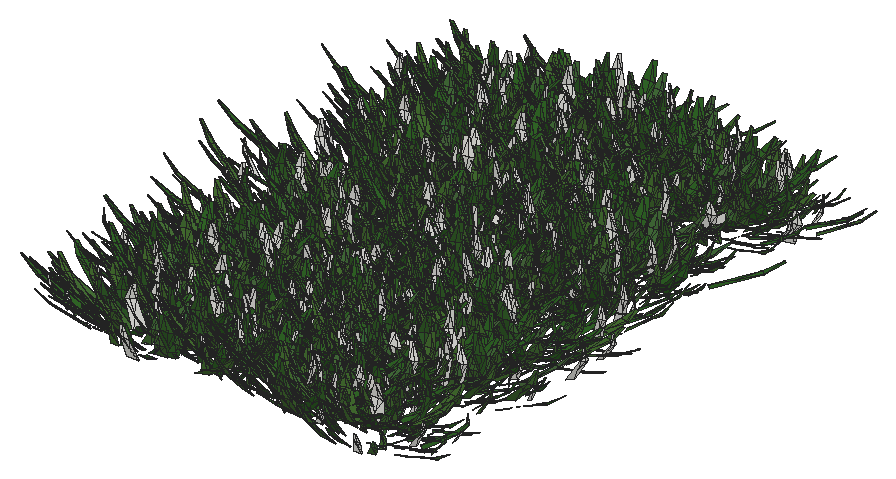
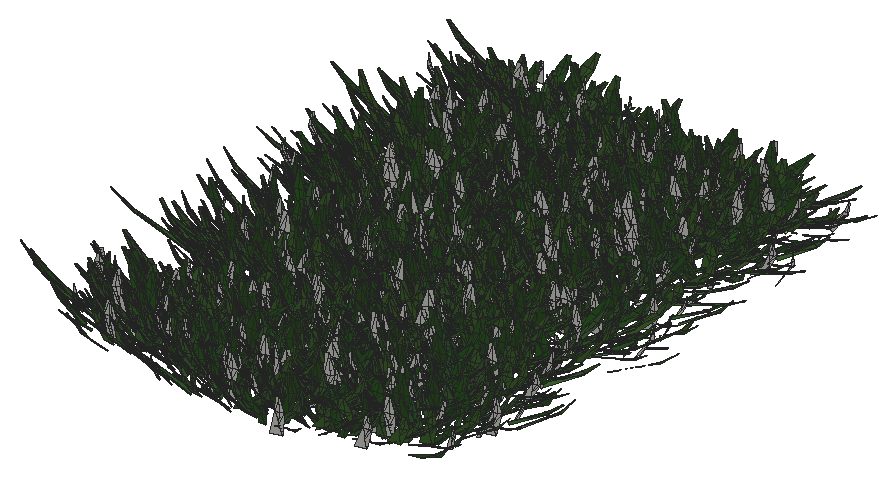
# SketchUp Ruby script. Lengths in inches.
U = 1.inch
M = Sketchup.active_model
def pt(a) = Geom::Point3d.new(a.map { |v| v * U })
def face(e, loops, mat)
  f = e.add_face(loops[0].map { |a| pt(a) })
  loops[1..].each { |l| e.add_face(l.map { |a| pt(a) }).erase! }
  f.material = f.back_material = mat if mat
  f
end
# faces: each face lists its corners as indices into pts; further lists are holes
def faces(e, pts, list, mat = nil) = list.each { |f| face(e, (f[0].is_a?(Array) ? f : [f]).map { |l| l.map { |i| pts[i] } }, mat) }
# xy, xz, yz: faces in a plane at the given z, y or x. An outline is a flat list of corners, or four numbers for a rectangle; further outlines are holes
def ring(l) = l.size == 4 ? [[l[0], l[1]], [l[2], l[1]], [l[2], l[3]], [l[0], l[3]]] : l.each_slice(2).to_a
def flat(e, list, mat, &to3) = list.each { |f| face(e, (f[0].is_a?(Array) ? f : [f]).map { |l| ring(l).map { |u, v| to3.(u, v) } }, mat) }
def xy(e, z, list, mat = nil) = flat(e, list, mat) { |x, y| [x, y, z] }
def xz(e, y, list, mat = nil) = flat(e, list, mat) { |x, z| [x, y, z] }
def yz(e, x, list, mat = nil) = flat(e, list, mat) { |y, z| [x, y, z] }
def lines(e, pts, list) = list.each { |a, b| e.add_line(pt(pts[a]), pt(pts[b])) }
# prism: a flat outline (further loops are holes) pulled along v
def prism(e, loops, v, mat = nil)
  f = face(e, loops, mat); d = Geom::Vector3d.new(v.map { |x| x * U })
  f.pushpull(f.normal.samedirection?(d) ? d.length : -d.length)
end
def box(e, o, s, mat = nil) = prism(e, [[o, [o[0] + s[0], o[1], o[2]], [o[0] + s[0], o[1] + s[1], o[2]], [o[0], o[1] + s[1], o[2]]]], [0, 0, s[2]], mat)
def at(x, y, z, deg = 0) = Geom::Transformation.translation(pt([x, y, z])) * Geom::Transformation.rotation(ORIGIN, Z_AXIS, deg.degrees)
def axes(o, x, y, z) = Geom::Transformation.new([*x, 0, *y, 0, *z, 0, *pt(o).to_a, 1])
def part(name) = M.definitions.add(name)
# library, detail: a bought-in or finely detailed component or shape, given as its bounding box
def library(name, o, s) = part(name).tap { |d| box(d.entities, o, s) }
def detail(e, o, s) = box(e.add_group.entities, o, s)
def put(e, d, t, mat = nil) = e.add_instance(d, t).tap { |i| i.material = mat if mat }
def group(e, t, mat = nil) = e.add_group.tap { |g| g.transformation = t; g.material = mat if mat }.entities
root = M.entities
M.materials.add("Material82").color = [68, 110, 58]
M.materials.add("Material83").color = [48, 90, 38]
M.materials.add("Material84").color = [68, 110, 48]
M.materials.add("Material85").color = [48, 90, 48]
M.materials.add("Material86").color = [58, 110, 58]
M.materials.add("Material87").color = [58, 90, 38]
M.materials.add("Material88").color = [68, 100, 58]
M.materials.add("Material89").color = [48, 100, 38]
c1 = part("grass00")
p = [[-0.6875,0.15,0],[-0.56,0.08,5.52],[-0.04,0.03,2.76],[0.48,-0.02,0],[0.35,-0.02,5.52],[-0.1,-0.14,5.52],
  [-0.12,0.65,8.37],[-0.42,0.65,8.37]]
faces(c1.entities,p,[[0,1,2,3],[3,2,4],[1,5,2],[5,4,2],[1,6,5],[4,5,6],[7,6,1]])
c2 = part("Group16\#1")
put(c2.entities,c1,axes([1.44,-0.61,-0.01],[0.05352,0.12609,0],[-0.10704,0.04543,0.07239],[0.06664,-0.02828,0.11628]),"Material85")
put(c2.entities,c1,axes([0.76,-0.15,-0.01],[0.04676,0.24062,0],[-0.23162,0.04501,0.06642],[0.0652,-0.01267,0.23595]),"Material82")
put(c2.entities,c1,axes([0.79,0.01,-0.01],[-0.00606,0.34651,0],[-0.34381,-0.00602,0.0432],[0.04319,0.00076,0.34386]))
put(c2.entities,c1,axes([1,0.23,-0.01],[-0.07192,0.31144,0],[-0.28722,-0.06632,0.1236],[0.12043,0.02781,0.29478]),"Material84")
put(c2.entities,c1,axes([1.66,0.77,-0.01],[-0.13828,0.29651,0],[-0.21551,-0.1005,0.22471],[0.20365,0.09498,0.23779]),"Material89")
put(c2.entities,c1,axes([0.6875,0.52,-0.01],[-0.18126,0.24051,0],[-0.22746,-0.17142,0.09788],[0.07817,0.05891,0.28481]),"Material84")
put(c2.entities,c1,axes([0.68,0.78,-0.01],[-0.215,0.18688,0],[-0.12385,-0.14248,0.21334],[0.13995,0.16101,0.18878]),"Material82")
put(c2.entities,c1,axes([0.56,1,-0.01],[-0.13756,0.07624,0],[-0.06159,-0.11112,0.0927],[0.04494,0.08108,0.12705]),"Material84")
put(c2.entities,c1,axes([0.2,0.64,-0.01],[-0.23729,0.07254,0],[-0.05711,-0.18681,0.153],[0.04473,0.14632,0.19535]),"Material89")
put(c2.entities,c1,axes([0.0625,0.72,-0.01],[-0.28874,0.02525,0],[-0.02179,-0.24916,0.14647],[0.01276,0.14591,0.25012]),"Material82")
put(c2.entities,c1,axes([-0.08,0.62,-0.01],[-0.34089,-0.04187,0],[0.03255,-0.26504,0.216],[-0.02633,0.21439,0.26703]),"Material89")
put(c2.entities,c1,axes([-0.34,0.98,-0.01],[-0.14314,-0.0493,0],[0.04397,-0.12769,0.06843],[-0.02228,0.0647,0.13505]),"Material89")
put(c2.entities,c1,axes([-0.87,1.45,-0.01],[-0.23488,-0.14114,0],[0.13761,-0.22901,0.06087],[-0.03135,0.05217,0.26717]))
put(c2.entities,c1,axes([-0.72,0.77,-0.01],[-0.14208,-0.13251,0],[0.07209,-0.0773,0.16301],[-0.11118,0.11922,0.1057]),"Material89")
put(c2.entities,c1,axes([-0.62,0.43,-0.01],[-0.14845,-0.21203,0],[0.18654,-0.13061,0.12304],[-0.10079,0.07057,0.22772]),"Material82")
put(c2.entities,c1,axes([-0.68,0.29,-0.01],[-0.13639,-0.32136,0],[0.31723,-0.13464,0.05579],[-0.05136,0.0218,0.34462]),"Material83")
put(c2.entities,c1,axes([-0.64,0.125,-0.01],[-0.0458,-0.23569,0],[0.22124,-0.043,0.08276],[-0.08124,0.01579,0.22538]),"Material86")
put(c2.entities,c1,axes([-1.6,-0.03,-0.01],[0.00576,-0.32897,0],[0.27526,0.00482,0.18018],[-0.18015,-0.00315,0.2753]),"Material84")
put(c2.entities,c1,axes([-1.36,-0.31,-0.01],[0.05718,-0.24765,0],[0.18172,0.04196,0.17267],[-0.16825,-0.03885,0.1865]),"Material89")
put(c2.entities,c1,axes([-1.54,-0.72,-0.01],[0.06537,-0.14017,0],[0.13555,0.06321,0.03939],[-0.0357,-0.01665,0.14956]))
put(c2.entities,c1,axes([-1.19,-0.9,-0.01],[0.09597,-0.12735,0],[0.11214,0.08451,0.07557],[-0.06035,-0.04548,0.14042]),"Material88")
put(c2.entities,c1,axes([-0.47,-0.54,-0.01],[0.11588,-0.10072,0],[0.0618,0.0711,0.12124],[-0.07953,-0.0915,0.0942]))
put(c2.entities,c1,axes([-0.47,-0.84,-0.01],[0.11927,-0.0661,0],[0.06603,0.11913,0.00646],[-0.00313,-0.00565,0.13621]),"Material84")
put(c2.entities,c1,axes([-0.38,-1.24,-0.01],[0.28037,-0.08571,0],[0.0618,0.20215,0.20315],[-0.05939,-0.19428,0.21139]),"Material88")
put(c2.entities,c1,axes([-0.06,-0.66,-0.01],[0.22719,-0.01987,0],[0.01247,0.14255,0.17758],[-0.01547,-0.17691,0.1431]),"Material87")
put(c2.entities,c1,axes([0.11,-0.89,-0.01],[0.14882,0.01828,0],[-0.01058,0.08611,0.12229],[0.01491,-0.12138,0.08676]),"Material85")
put(c2.entities,c1,axes([0.25,-0.72,-0.01],[0.20481,0.07053,0],[-0.06206,0.18022,0.10291],[0.03351,-0.0973,0.1906]),"Material85")
put(c2.entities,c1,axes([0.85,-1.42,-0.01],[0.16481,0.09904,0],[-0.09472,0.15762,0.05616],[0.02893,-0.04814,0.18389]),"Material84")
put(c2.entities,c1,axes([1.01,-1.09,-0.01],[0.21858,0.20385,0],[-0.17495,0.1876,0.15339],[0.10462,-0.11218,0.25652]),"Material89")
put(c2.entities,c1,axes([1.01,-0.71,-0.01],[0.08733,0.12473,0],[-0.06445,0.04512,0.13037],[0.1068,-0.07477,0.07867]),"Material85")
c3 = part("Group15\#1")
put(c3.entities,c2,at(0,0,0))
c4 = part("3darcstudiotree_grass00\#1")
put(c4.entities,c3,at(0,0,0))
put(root,c4,axes([1764.47,953.26,-29.74],[1.08587,1.67228,0],[-4.264,0.43062,-0.00469],[-0.02209,0.00223,1.60422]))
put(root,c4,axes([1765.97,973.1875,-29.74],[-3.39635,0.60304,0],[-1.8174,-1.59194,-0.05685],[-0.1325,-0.11606,1.88376]))
put(root,c4,axes([1765.31,943.77,-29.74],[-0.8053,1.43922,0],[-4.1788,-0.36366,-0.05256],[-0.20936,-0.01822,1.30827]))
put(root,c4,axes([1766.12,990.89,-29.74],[1.7154,-1.15643,0],[3.09768,0.71465,-0.02347],[0.14538,0.03354,1.9305]))
put(root,c4,axes([1766.8,971.14,-29.74],[-0.55616,-1.38612,0],[4.6364,-0.28933,-0.05346],[0.22148,-0.01382,1.47567]))
put(root,c4,axes([1766.16,949.59,-29.74],[2.313,-1.43442,0],[2.99954,0.75225,-0.04064],[0.1888,0.04735,1.46692]))
put(root,c4,axes([1766.23,988.37,-29.74],[2.50193,-0.87133,0],[2.32937,1.04026,-0.01409],[0.05813,0.02596,1.64399]))
put(root,c4,axes([1766.46,958.98,-29.74],[2.27709,-1.12887,0],[2.96357,0.92974,-0.01848],[0.07518,0.02359,1.47553]))
put(root,c4,axes([1765.4,986.68,-29.74],[4.07348,0.57799,0],[-1.18057,1.29405,-0.01256],[-0.02962,0.03247,1.82155]))
put(root,c4,axes([1765.55,969.1,-29.74],[2.25028,1.20461,0],[-3.26486,0.94856,-0.0323],[-0.12798,0.03718,1.496]))
put(root,c4,axes([1766.18,980.93,-29.74],[-1.39977,1.36626,0],[-3.55438,-0.56636,-0.02451],[-0.1313,-0.02092,1.66036]))
put(root,c4,axes([1765.67,950.59,-29.74],[3.43029,0.99275,0],[-1.97308,1.06035,-0.01519],[-0.04853,0.02608,1.34969]))
put(root,c4,axes([1766.625,946.78,-29.74],[-1.21632,1.56365,0],[-3.36368,-0.40694,-0.03727],[-0.21338,-0.02582,1.57911]))
put(root,c4,axes([1766,963.77,-29.74],[4.01997,0.45296,0],[-1.05214,1.45226,-0.01128],[-0.01738,0.02399,1.61003]))
put(root,c4,axes([1766.32,966.45,-29.74],[4.2861,-0.44175,0],[0.90749,1.36943,-0.02428],[0.0455,0.06867,1.99391]))
put(root,c4,axes([1766.625,983.88,-29.74],[3.51248,0.23364,0],[-0.65189,1.52422,-0.03005],[-0.02625,0.06139,1.54341]))
put(root,c4,axes([1767.13,942.05,-29.74],[3.31562,-0.63662,0],[1.81859,1.47309,-0.02466],[0.05194,0.04207,1.49812]))
put(root,c4,axes([1767.43,977.47,-29.74],[-0.84571,1.33613,0],[-3.59715,-0.35412,-0.00012],[-0.00056,-0.00006,1.39497]))
put(root,c4,axes([1767.76,992.93,-29.74],[-1.51727,1.49458,0],[-3.30202,-0.52136,-0.01826],[-0.09361,-0.01478,1.47196]))
put(root,c4,axes([1768.125,955.89,-29.74],[3.22727,-0.96219,0],[2.40393,1.25403,-0.04167],[0.15655,0.08166,1.86151]))
put(root,c4,axes([1769.59,953.09,-29.74],[-3.43052,-0.93956,0],[2.00829,-1.14045,-0.00375],[0.01479,-0.0084,1.82358]))
put(root,c4,axes([1769.65,946.7,-29.74],[-2.79747,-0.82267,0],[2.4,-1.26929,-0.00029],[0.00098,-0.00052,1.69542]))
put(root,c4,axes([1768.03,980.14,-29.74],[3.76479,0.94059,0],[-2.16386,1.34705,-0.03414],[-0.08584,0.05343,1.42377]))
put(root,c4,axes([1769.74,960.45,-29.74],[-3.74102,0.70585,0],[-1.92999,-1.5909,-0.05113],[-0.08819,-0.0727,1.33965]))
put(root,c4,axes([1770.01,982.32,-29.74],[2.94171,-1.11183,0],[3.18535,1.31078,-0.03986],[0.13301,0.05473,1.66404]))
put(root,c4,axes([1770.49,941.6875,-29.74],[-3.65106,0.9561,0],[-2.55118,-1.5152,-0.05111],[-0.12576,-0.07469,1.53759]))
put(root,c4,axes([1770.46,968.48,-29.74],[-2.1448,1.18286,0],[-3.37437,-0.95161,-0.05929],[-0.21963,-0.06194,1.41608]))
put(root,c4,axes([1769.625,951.12,-29.74],[2.61816,1.29298,0],[-2.60516,0.82044,-0.01421],[-0.06264,0.01973,1.40932]))
put(root,c4,axes([1771.41,983.85,-29.74],[-0.23596,-1.70659,0],[3.32039,-0.0714,-0.01049],[0.06174,-0.00133,1.4693]))
put(root,c4,axes([1772.3125,985.85,-29.74],[-2.68837,-0.8629,0],[2.90522,-1.40773,-0.04334],[0.1065,-0.05161,1.34295]))
put(root,c4,axes([1771.64,980.02,-29.74],[2.30193,-1.12166,0],[3.41965,1.0915,-0.0352],[0.15447,0.0493,1.86157]))
put(root,c4,axes([1772.61,977.03,-29.74],[-3.8851,-1.03716,0],[2.44189,-1.42264,-0.04034],[0.11257,-0.06558,1.62559]))
put(root,c4,axes([1770.54,957.93,-29.74],[4.25337,0.6683,0],[-1.56461,1.54873,-0.01606],[-0.02903,0.02874,1.54782]))
put(root,c4,axes([1770.84,975.2,-29.74],[0.91536,1.26151,0],[-4.37209,0.4934,-0.02742],[-0.14974,0.0169,1.93645]))
put(root,c4,axes([1771.09,966.12,-29.74],[-0.09975,1.34747,0],[-4.08432,-0.04703,-0.00454],[-0.02466,-0.00028,1.66362]))
put(root,c4,axes([1773.08,964.17,-29.74],[-1.28823,-1.73919,0],[3.44626,-0.39701,-0.03009],[0.18497,-0.02131,1.72353]))
put(root,c4,axes([1771.98,995.19,-29.74],[3.82297,0.44431,0],[-0.93883,1.25636,-0.026],[-0.04711,0.06304,1.59572]))
put(root,c4,axes([1773.51,991.98,-29.74],[1.61408,-1.6002,0],[4.35972,0.68394,-0.04298],[0.19186,0.0301,1.68954]))
put(root,c4,axes([1772.17,989.56,-29.74],[4.08766,0.51132,0],[-1.24704,1.55051,-0.00141],[-0.00269,0.00335,1.95289]))
put(root,c4,axes([1772.65,944.97,-29.74],[0.40934,1.39565,0],[-3.638,0.16595,-0.04522],[-0.26335,0.01201,1.60941]))
put(root,c4,axes([1773.06,949.33,-29.74],[-2.97215,1.15542,0],[-3.15373,-1.26173,-0.01243],[-0.04576,-0.01831,1.76595]))
put(root,c4,axes([1773.07,987.72,-29.74],[4.03922,-0.03156,0],[0.07296,1.45219,-0.01855],[0.00258,0.0513,1.93628]))
put(root,c4,axes([1773.16,955.45,-29.74],[1.39622,1.62786,0],[-3.6301,0.48424,-0.04556],[-0.23124,0.03085,1.53888]))
put(root,c4,axes([1773.66,961.14,-29.74],[4.28281,-0.63976,0],[1.42181,1.48036,-0.01068],[0.01649,0.01717,1.31138]))
put(root,c4,axes([1773.62,973.6,-29.74],[3.35774,0.54146,0],[-1.57719,1.52117,-0.03911],[-0.07127,0.06874,1.50402]))
put(root,c4,axes([1775.55,964.76,-29.74],[-1.97401,-1.44609,0],[3.51216,-0.74566,-0.02018],[0.11603,-0.02463,1.95264]))
put(root,c4,axes([1775.49,979.34,-29.74],[-2.39621,-0.97294,0],[2.61152,-1.00033,-0.02073],[0.08443,-0.03234,1.5494]))
put(root,c4,axes([1773.54,970.62,-29.74],[2.01516,1.65729,0],[-3.55056,0.67146,-0.00104],[-0.005,0.00095,1.58037]))
put(root,c4,axes([1776.04,976.84,-29.74],[-3.41262,-0.98405,0],[2.00346,-1.0806,-0.03203],[0.14502,-0.07822,1.95145]))
put(root,c4,axes([1775.22,942.67,-29.74],[3.35024,-0.43777,0],[1.10858,1.31952,-0.03222],[0.06859,0.08164,1.78787]))
put(root,c4,axes([1775.86,994.33,-29.74],[2.23301,-1.20393,0],[2.80312,0.80861,-0.02877],[0.133,0.03837,1.49076]))
put(root,c4,axes([1777.32,973.25,-29.74],[-1.89614,-1.52378,0],[3.69892,-0.71587,-0.01008],[0.04587,-0.00888,1.566]))
put(root,c4,axes([1775.73,946.05,-29.74],[0.10079,1.33733,0],[-4.05045,0.04748,-0.05613],[-0.28184,0.0033,1.5259]))
put(root,c4,axes([1776.44,967.75,-29.74],[3.01451,-0.88182,0],[2.30556,1.22582,-0.02804],[0.08966,0.04767,1.55696]))
put(root,c4,axes([1775.67,945.2,-29.74],[2.52987,0.96809,0],[-2.35442,0.95693,-0.00683],[-0.03278,0.01332,1.74693]))
put(root,c4,axes([1777.19,990.53,-29.74],[-4.40755,0.3662,0],[-0.80873,-1.51388,-0.00142],[-0.00162,-0.00303,1.63114]))
put(root,c4,axes([1777.46,970.07,-29.74],[-3.86461,-0.59074,0],[1.45311,-1.4785,-0.05586],[0.12869,-0.13094,1.92103]))
put(root,c4,axes([1777.59,954.54,-29.74],[0.04452,-1.40138,0],[3.5701,0.01764,-0.00992],[0.04898,0.00024,1.32167]))
put(root,c4,axes([1777.3125,992.66,-29.74],[-3.74567,1.07998,0],[-2.52019,-1.35944,-0.03994],[-0.14532,-0.07839,1.97331]))
put(root,c4,axes([1776.27,985.13,-29.74],[4.59378,0.22046,0],[-0.54654,1.77125,-0.0359],[-0.02405,0.07793,1.88046]))
put(root,c4,axes([1777.61,980.81,-29.74],[1.47145,-1.32607,0],[3.01918,0.52105,-0.00213],[0.01031,0.00178,1.30651]))
put(root,c4,axes([1778.73,948.32,-29.74],[-2.64283,-1.13535,0],[3.48014,-1.25993,-0.02326],[0.08818,-0.03192,1.82249]))
put(root,c4,axes([1778.1875,951.53,-29.74],[1.26532,-1.44178,0],[3.12553,0.42661,-0.00044],[0.00223,0.0003,1.32507]))
put(root,c4,axes([1778.71,961.61,-29.74],[-4.13794,-0.2249,0],[0.58111,-1.66288,-0.00876],[0.00496,-0.01418,1.32289]))
put(root,c4,axes([1777.75,983.75,-29.74],[-2.89048,1.44179,0],[-2.90546,-0.90593,-0.0043],[-0.02277,-0.0071,1.8735]))
put(root,c4,axes([1776.85,975.54,-29.74],[2.24895,1.38406,0],[-3.92977,0.99312,-0.02786],[-0.13256,0.0335,1.9768]))
put(root,c4,axes([1777.81,952.74,-29.74],[3.40614,0.32781,0],[-0.81542,1.31776,-0.01459],[-0.02356,0.03807,1.75568]))
put(root,c4,axes([1777.88,996.99,-29.74],[4.11101,0.00408,0],[-0.01055,1.6533,-0.01268],[-0.00019,0.02913,1.83013]))
put(root,c4,axes([1778.03,988.6875,-29.74],[4.61322,-0.12203,0],[0.30512,1.79396,-0.00473],[0.00139,0.00815,1.49489]))
put(root,c4,axes([1777.94,957.56,-29.74],[3.60093,0.62069,0],[-1.54425,1.39338,-0.01451],[-0.03218,0.02903,1.59989]))
put(root,c4,axes([1779.04,960.13,-29.74],[-0.93158,1.57452,0],[-3.64716,-0.33561,-0.02125],[-0.09909,-0.00912,1.34411]))
put(root,c4,axes([1778.92,965.66,-29.74],[1.53583,1.49996,0],[-3.93703,0.62697,-0.05886],[-0.22971,0.03658,1.33951]))
put(root,c4,axes([1781.17,959.57,-29.74],[-2.29669,-1.11112,0],[2.95834,-0.95105,-0.00371],[0.01505,-0.00484,1.4993]))
put(root,c4,axes([1781.1,994.95,-29.74],[-2.49297,-0.95003,0],[2.84759,-1.16217,-0.03177],[0.13042,-0.05323,1.8145]))
put(root,c4,axes([1780.91,965.81,-29.74],[-2.8718,1.45727,0],[-2.81901,-0.86401,-0.03149],[-0.12433,-0.03811,1.33797]))
put(root,c4,axes([1780.86,957.45,-29.74],[-2.73949,1.39402,0],[-3.69271,-1.12865,-0.03455],[-0.12332,-0.03769,1.58129]))
put(root,c4,axes([1782.3,985.67,-29.74],[-2.79426,-0.70511,0],[1.77672,-1.09506,-0.02395],[0.07288,-0.04492,1.39534]))
put(root,c4,axes([1781.11,948.12,-29.74],[4.32757,-0.42653,0],[1.12297,1.77206,-0.03338],[0.0321,0.05066,1.37691]))
put(root,c4,axes([1781.38,974.3,-29.74],[3.39282,-0.2362,0],[0.75884,1.6953,-0.03701],[0.03902,0.08718,1.98432]))
put(root,c4,axes([1781.33,983.04,-29.74],[1.01985,1.24994,0],[-3.27441,0.41552,-0.0339],[-0.22651,0.02874,1.80984]))
put(root,c4,axes([1781.78,955.09,-29.74],[3.17214,0.39156,0],[-1.05658,1.33127,-0.01935],[-0.04192,0.05282,1.92273]))
put(root,c4,axes([1782.09,972.06,-29.74],[3.44047,-0.2055,0],[0.68194,1.77564,-0.05863],[0.04271,0.1112,1.66018]))
put(root,c4,axes([1782.9,992.99,-29.74],[-2.53173,1.21264,0],[-2.8931,-0.93942,-0.04557],[-0.23211,-0.07537,1.85346]))
put(root,c4,axes([1783.66,946.88,-29.74],[-3.83423,-0.51133,0],[1.38691,-1.61748,-0.06149],[0.1095,-0.1277,1.80385]))
put(root,c4,axes([1783.76,971.34,-29.74],[-2.06404,-1.37727,0],[3.69374,-0.86095,-0.04139],[0.20463,-0.0477,1.84708]))
put(root,c4,axes([1781.96,981.04,-29.74],[2.13019,1.09948,0],[-3.08878,0.93074,-0.0123],[-0.05365,0.01617,1.59876]))
put(root,c4,axes([1784.04,987.38,-29.74],[-4.29389,-0.13256,0],[0.34176,-1.72178,-0.05117],[0.01874,-0.09441,1.54048]))
put(root,c4,axes([1782.67,942.03,-29.74],[4.09444,0.12503,0],[-0.31641,1.61154,-0.0417],[-0.02006,0.10219,1.91485]))
put(root,c4,axes([1784.03,967.74,-29.74],[-3.97452,0.57658,0],[-1.26948,-1.361,-0.04924],[-0.12234,-0.13116,1.98345]))
put(root,c4,axes([1782.76,979.83,-29.74],[4.64305,-0.03413,0],[0.08366,1.7702,-0.03615],[0.00311,0.0658,1.55355]))
put(root,c4,axes([1782.6,944.35,-29.74],[3.61655,0.77067,0],[-2.16585,1.58076,-0.05913],[-0.11484,0.08382,1.39517]))
put(root,c4,axes([1784.02,950.95,-29.74],[-3.45507,0.18922,0],[-0.60525,-1.7188,-0.02154],[-0.01288,-0.03658,1.4342]))
put(root,c4,axes([1784.41,996.36,-29.74],[-3.18702,-0.48311,0],[1.45771,-1.49562,-0.04802],[0.08757,-0.08985,1.54794]))
put(root,c4,axes([1783.4,952.61,-29.74],[1.33968,1.52005,0],[-3.16755,0.43419,-0.01128],[-0.07711,0.01057,1.81963]))
put(root,c4,axes([1783.97,962.625,-29.74],[-0.83712,1.35251,0],[-3.5635,-0.34303,-0.03757],[-0.17469,-0.01682,1.3158]))
put(root,c4,axes([1784.73,964.89,-29.74],[3.08356,-0.59749,0],[1.85245,1.48689,-0.05746],[0.15906,0.12767,1.97658]))
put(root,c4,axes([1784.62,977.9,-29.74],[1.55645,1.18195,0],[-3.2541,0.66647,-0.04821],[-0.21297,0.04362,1.36797]))
put(root,c4,axes([1784.76,990.47,-29.74],[0.845,1.27042,0],[-4.02841,0.41673,-0.05161],[-0.24313,0.02515,1.52021]))
put(root,c4,axes([1786.95,970.42,-29.74],[-3.70591,-0.99796,0],[1.87776,-1.08451,-0.01838],[0.07513,-0.04339,1.80866]))
put(root,c4,axes([1786.98,986.51,-29.74],[0.0983,-1.39772,0],[3.56781,0.03903,-0.00183],[0.01012,0.00011,1.48199]))
put(root,c4,axes([1786.66,951.6875,-29.74],[2.17735,-1.14497,0],[3.55677,1.05197,-0.03529],[0.11494,0.03399,1.35654]))
put(root,c4,axes([1787.6,964.24,-29.74],[-4.087,-0.33484,0],[0.93219,-1.7696,-0.02537],[0.02744,-0.05209,1.82613]))
put(root,c4,axes([1787.26,975.18,-29.74],[-3.8828,0.51827,0],[-1.09306,-1.27365,-0.02484],[-0.06133,-0.07146,1.96802]))
put(root,c4,axes([1787.54,955.43,-29.74],[-4.01589,0.275,0],[-0.74615,-1.69466,-0.05401],[-0.03733,-0.08478,1.3206]))
put(root,c4,axes([1786.98,960.24,-29.74],[-1.92395,1.11114,0],[-2.73961,-0.73778,-0.01899],[-0.11099,-0.02989,1.75992]))
put(root,c4,axes([1786.32,941.76,-29.74],[-0.14266,1.36173,0],[-4.10184,-0.06683,-0.00296],[-0.01424,-0.00023,1.47961]))
put(root,c4,axes([1786.58,965.58,-29.74],[-0.37072,1.84099,0],[-4.27519,-0.13389,-0.01448],[-0.06545,-0.00205,1.45727]))
put(root,c4,axes([1786.79,994.4,-29.74],[4.18586,0.29447,0],[-0.62505,1.38186,-0.04495],[-0.05854,0.12943,1.97854]))
put(root,c4,axes([1788.87,967.85,-29.74],[-0.69027,-1.34957,0],[4.18043,-0.33255,-0.04603],[0.23408,-0.01862,1.65834]))
put(root,c4,axes([1787.48,943.8,-29.74],[3.68364,0.44666,0],[-1.28613,1.64968,-0.02064],[-0.02718,0.03487,1.46981]))
put(root,c4,axes([1788.82,981.01,-29.74],[-3.79382,0.9598,0],[-2.14839,-1.32076,-0.01729],[-0.051,-0.03135,1.62898]))
put(root,c4,axes([1789.47,952.49,-29.74],[-3.50392,-0.27669,0],[0.88512,-1.7433,-0.02406],[0.02146,-0.04227,1.53532]))
put(root,c4,axes([1789.74,988.08,-29.74],[-4.49069,-0.28234,0],[0.61208,-1.5141,-0.05098],[0.04605,-0.11392,1.67187]))
put(root,c4,axes([1788.29,977.58,-29.74],[4.2001,-0.13479,0],[0.33266,1.61217,-0.01977],[0.00834,0.04041,1.59866]))
put(root,c4,axes([1789.56,979.17,-29.74],[-4.51566,0.3438,0],[-0.75132,-1.53478,-0.00152],[-0.00137,-0.0028,1.41339]))
put(root,c4,axes([1788.5,972,-29.74],[-1.23007,1.60855,0],[-3.72331,-0.44283,-0.01363],[-0.06328,-0.00753,1.41312]))
put(root,c4,axes([1789.1875,946.86,-29.74],[-2.10873,0.99525,0],[-2.92476,-0.96381,-0.03387],[-0.14037,-0.04626,1.54303]))
put(root,c4,axes([1789.03,949.03,-29.74],[3.33633,-0.58263,0],[1.85643,1.65335,-0.04981],[0.10311,0.09183,1.75709]))
put(root,c4,axes([1788.71,983.75,-29.74],[2.36553,1.18037,0],[-3.06807,0.95629,-0.02315],[-0.10187,0.03175,1.64391]))
put(root,c4,axes([1788.59,992.54,-29.74],[2.70315,0.92974,0],[-3.09727,1.40055,-0.01764],[-0.05733,0.02592,1.74631]))
put(root,c4,axes([1789.88,961.79,-29.74],[2.84805,-1.35819,0],[2.78081,0.90692,-0.04304],[0.21584,0.07039,1.76026]))
put(root,c4,axes([1789.33,956.85,-29.74],[0.25957,1.50579,0],[-3.94932,0.10588,-0.02807],[-0.1244,0.00334,1.3177]))
put(root,c4,axes([1791.9375,942.74,-29.74],[-2.56709,-0.87628,0],[2.75862,-1.25691,-0.00422],[0.01164,-0.0053,1.33295]))
put(root,c4,axes([1790.22,990.16,-29.74],[3.46346,0.58344,0],[-1.61207,1.48838,-0.00364],[-0.00911,0.00841,1.96053]))
put(root,c4,axes([1793.0625,988.43,-29.74],[-2.62594,-1.45094,0],[3.42478,-0.964,-0.01802],[0.06257,-0.01761,1.345]))
put(root,c4,axes([1792.57,979.68,-29.74],[-3.57945,0.04189,0],[-0.11544,-1.5341,-0.02538],[-0.0045,-0.05977,1.74242]))
put(root,c4,axes([1791.84,957.48,-29.74],[-2.10864,1.34219,0],[-3.56504,-0.87109,-0.01218],[-0.05259,-0.01285,1.59607]))
put(root,c4,axes([1792.54,951.41,-29.74],[3.4734,-0.75241,0],[2.06047,1.47936,-0.02691],[0.07219,0.05183,1.78778]))
put(root,c4,axes([1793.82,944.38,-29.74],[-1.56362,-1.21345,0],[3.6466,-0.73082,-0.00876],[0.03709,-0.00743,1.45672]))
put(root,c4,axes([1794.05,959.59,-29.74],[-3.17921,-1.35137,0],[3.1644,-1.15784,-0.01209],[0.04457,-0.01631,1.62724]))
put(root,c4,axes([1794.12,963.76,-29.74],[-2.5712,-1.27561,0],[3.33499,-1.0455,-0.01168],[0.0385,-0.01207,1.34439]))
put(root,c4,axes([1792.43,974.79,-29.74],[-0.16089,1.57179,0],[-4.27524,-0.06806,-0.04298],[-0.25282,-0.00402,1.88799]))
put(root,c4,axes([1794.17,968.13,-29.74],[-3.47552,-0.34069,0],[1.08655,-1.72393,-0.01735],[0.02109,-0.03347,1.70162]))
put(root,c4,axes([1794.08,971.25,-29.74],[-3.29266,-0.34854,0],[0.95777,-1.40726,-0.03217],[0.05606,-0.08237,1.86146]))
put(root,c4,axes([1792.31,949.47,-29.74],[2.09092,1.38555,0],[-3.43654,0.80658,-0.00188],[-0.01015,0.00238,1.87843]))
put(root,c4,axes([1792.71,972.92,-29.74],[1.95292,1.06951,0],[-2.86765,0.8144,-0.02117],[-0.10996,0.03123,1.69559]))
put(root,c4,axes([1793.38,961.49,-29.74],[-1.97289,1.32597,0],[-3.97358,-0.91953,-0.01374],[-0.05147,-0.01191,1.50009]))
put(root,c4,axes([1793.02,940.58,-29.74],[0.75696,1.65896,0],[-4.64105,0.32936,-0.03105],[-0.12997,0.00922,1.50318]))
put(root,c4,axes([1793.21,977.4,-29.74],[4.5376,0.13529,0],[-0.33368,1.74059,-0.04634],[-0.02094,0.10925,1.98901]))
put(root,c4,axes([1793.35,986.54,-29.74],[1.35175,1.46561,0],[-4.38115,0.62846,-0.0524],[-0.19286,0.02766,1.36852]))
put(root,c4,axes([1795.24,990.7,-29.74],[-4.23196,-0.66829,0],[1.43136,-1.40974,-0.04264],[0.09281,-0.09141,1.69007]))
put(root,c4,axes([1794.26,993.125,-29.74],[2.88826,-0.72218,0],[1.92215,1.1956,-0.03299],[0.1167,0.07259,1.77748]))
put(root,c4,axes([1794.84,953.89,-29.74],[-2.97303,0.61552,0],[-2.04085,-1.53313,-0.02543],[-0.06857,-0.05151,1.9093]))
put(root,c4,axes([1794.12,994.58,-29.74],[1.93247,1.08024,0],[-2.71059,0.75417,-0.03223],[-0.14585,0.04058,1.37708]))
